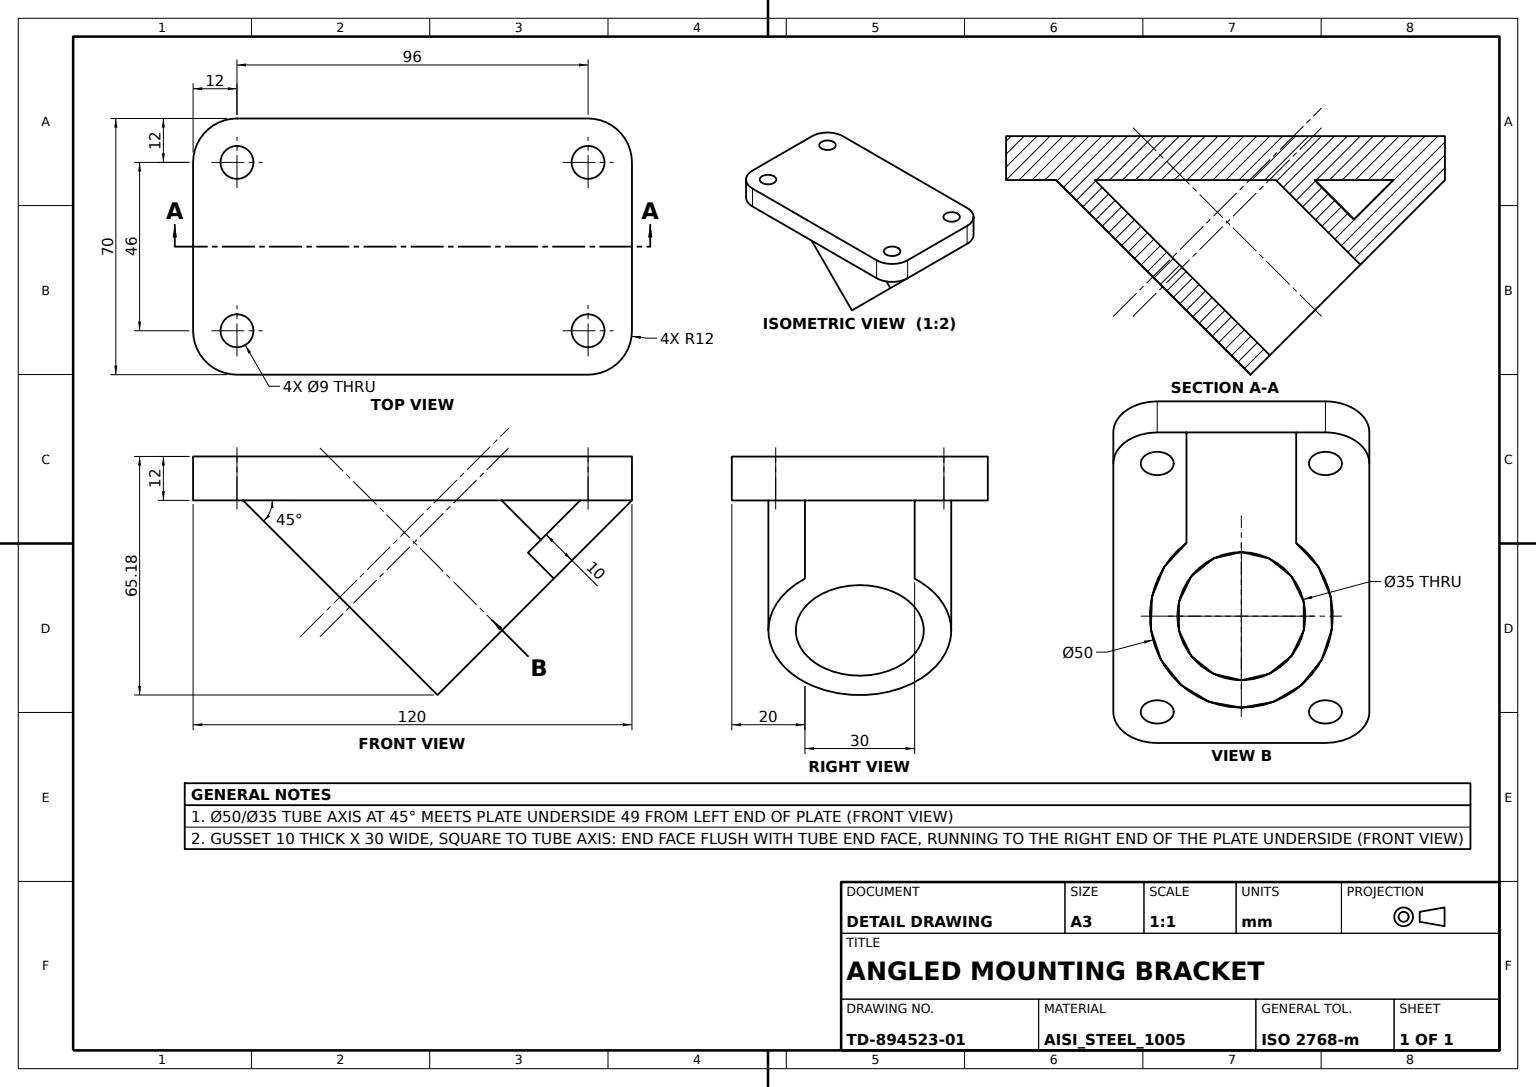
ISO-10303-21;
HEADER;
FILE_DESCRIPTION((''),'2;1');
FILE_NAME('','',(''),(''),'','','');
FILE_SCHEMA(('AUTOMOTIVE_DESIGN'));
ENDSEC;
DATA;
#1=APPLICATION_CONTEXT('');
#2=PRODUCT_CONTEXT('',#1,'mechanical');
#3=PRODUCT('','','',(#2));
#4=PRODUCT_DEFINITION_FORMATION('','',#3);
#5=PRODUCT_DEFINITION_CONTEXT('',#1,'design');
#6=PRODUCT_DEFINITION('','',#4,#5);
#7=PRODUCT_DEFINITION_SHAPE('','',#6);
#8=(LENGTH_UNIT()NAMED_UNIT(*)SI_UNIT(.MILLI.,.METRE.));
#9=(NAMED_UNIT(*)PLANE_ANGLE_UNIT()SI_UNIT($,.RADIAN.));
#10=(NAMED_UNIT(*)SI_UNIT($,.STERADIAN.)SOLID_ANGLE_UNIT());
#11=UNCERTAINTY_MEASURE_WITH_UNIT(LENGTH_MEASURE(0.005),#8,'distance_accuracy_value','');
#12=(GEOMETRIC_REPRESENTATION_CONTEXT(3)GLOBAL_UNCERTAINTY_ASSIGNED_CONTEXT((#11))GLOBAL_UNIT_ASSIGNED_CONTEXT((#8,#9,#10))REPRESENTATION_CONTEXT('',''));
#13=CARTESIAN_POINT('',(-50.,120.,0.));
#14=VERTEX_POINT('',#13);
#15=CARTESIAN_POINT('',(-50.,105.857864,0.));
#16=VERTEX_POINT('',#15);
#17=CARTESIAN_POINT('',(-50.,0.,0.));
#18=DIRECTION('',(0.,-1.,0.));
#19=VECTOR('',#18,1000.);
#20=LINE('',#17,#19);
#21=EDGE_CURVE('',#14,#16,#20,.T.);
#22=ORIENTED_EDGE('',*,*,#21,.F.);
#23=CARTESIAN_POINT('',(-50.,98.642136,-21.357864));
#24=VERTEX_POINT('',#23);
#25=DIRECTION('',(0.,-0.707106781,-0.707106781));
#26=VECTOR('',#25,1000.);
#27=LINE('',#13,#26);
#28=EDGE_CURVE('',#14,#24,#27,.T.);
#29=ORIENTED_EDGE('',*,*,#28,.T.);
#30=CARTESIAN_POINT('',(-50.,91.571068,-14.286797));
#31=VERTEX_POINT('',#30);
#32=CARTESIAN_POINT('',(-50.,26.042136,51.242136));
#33=DIRECTION('',(0.,0.707106781,-0.707106781));
#34=VECTOR('',#33,1000.);
#35=LINE('',#32,#34);
#36=EDGE_CURVE('',#31,#24,#35,.T.);
#37=ORIENTED_EDGE('',*,*,#36,.F.);
#38=CARTESIAN_POINT('',(-50.,112.928932,7.071068));
#39=LINE('',#38,#26);
#40=EDGE_CURVE('',#16,#31,#39,.T.);
#41=ORIENTED_EDGE('',*,*,#40,.F.);
#42=EDGE_LOOP('',(#22,#29,#37,#41));
#43=FACE_BOUND('',#42,.T.);
#44=DIRECTION('',(1.,0.,0.));
#45=DIRECTION('',(0.,0.,-1.));
#46=AXIS2_PLACEMENT_3D('',#38,#44,#45);
#47=PLANE('',#46);
#48=ADVANCED_FACE('',(#43),#47,.F.);
#49=CARTESIAN_POINT('',(-20.,120.,0.));
#50=VERTEX_POINT('',#49);
#51=DIRECTION('',(-1.,0.,0.));
#52=VECTOR('',#51,1000.);
#53=LINE('',#49,#52);
#54=EDGE_CURVE('',#50,#14,#53,.T.);
#55=ORIENTED_EDGE('',*,*,#54,.F.);
#56=CARTESIAN_POINT('',(-20.,98.642136,-21.357864));
#57=VERTEX_POINT('',#56);
#58=CARTESIAN_POINT('',(-20.,97.739823,-22.260177));
#59=DIRECTION('',(0.,0.707106781,0.707106781));
#60=VECTOR('',#59,1000.);
#61=LINE('',#58,#60);
#62=EDGE_CURVE('',#57,#50,#61,.T.);
#63=ORIENTED_EDGE('',*,*,#62,.F.);
#64=CARTESIAN_POINT('',(-35.,84.5,-35.5));
#65=AXIS2_PLACEMENT_3D('',#64,#33,#44);
#66=CIRCLE('',#65,25.);
#67=EDGE_CURVE('',#57,#24,#66,.T.);
#68=ORIENTED_EDGE('',*,*,#67,.T.);
#69=ORIENTED_EDGE('',*,*,#28,.F.);
#70=EDGE_LOOP('',(#55,#63,#68,#69));
#71=FACE_BOUND('',#70,.T.);
#72=CARTESIAN_POINT('',(-17.5,84.5,-35.5));
#73=VERTEX_POINT('',#72);
#74=CIRCLE('',#65,17.5);
#75=EDGE_CURVE('',#73,#73,#74,.T.);
#76=ORIENTED_EDGE('',*,*,#75,.F.);
#77=EDGE_LOOP('',(#76));
#78=FACE_BOUND('',#77,.T.);
#79=AXIS2_PLACEMENT_3D('',#64,#33,#59);
#80=PLANE('',#79);
#81=ADVANCED_FACE('',(#71,#78),#80,.T.);
#82=CARTESIAN_POINT('',(-20.,91.571068,-14.286797));
#83=VERTEX_POINT('',#82);
#84=CARTESIAN_POINT('',(-20.,105.857864,0.));
#85=VERTEX_POINT('',#84);
#86=CARTESIAN_POINT('',(-20.,90.668755,-15.18911));
#87=LINE('',#86,#60);
#88=EDGE_CURVE('',#83,#85,#87,.T.);
#89=ORIENTED_EDGE('',*,*,#88,.F.);
#90=CARTESIAN_POINT('',(-20.,26.042136,51.242136));
#91=LINE('',#90,#34);
#92=EDGE_CURVE('',#57,#83,#91,.F.);
#93=ORIENTED_EDGE('',*,*,#92,.F.);
#94=ORIENTED_EDGE('',*,*,#62,.T.);
#95=CARTESIAN_POINT('',(-20.,0.,0.));
#96=DIRECTION('',(0.,1.,0.));
#97=VECTOR('',#96,1000.);
#98=LINE('',#95,#97);
#99=EDGE_CURVE('',#85,#50,#98,.T.);
#100=ORIENTED_EDGE('',*,*,#99,.F.);
#101=EDGE_LOOP('',(#89,#93,#94,#100));
#102=FACE_BOUND('',#101,.T.);
#103=DIRECTION('',(0.,0.,1.));
#104=AXIS2_PLACEMENT_3D('',#86,#51,#103);
#105=PLANE('',#104);
#106=ADVANCED_FACE('',(#102),#105,.F.);
#107=CARTESIAN_POINT('',(-16.5,12.,12.));
#108=VERTEX_POINT('',#107);
#109=CARTESIAN_POINT('',(-12.,12.,12.));
#110=AXIS2_PLACEMENT_3D('',#109,#45,#51);
#111=CIRCLE('',#110,4.5);
#112=EDGE_CURVE('',#108,#108,#111,.T.);
#113=ORIENTED_EDGE('',*,*,#112,.T.);
#114=EDGE_LOOP('',(#113));
#115=FACE_BOUND('',#114,.T.);
#116=CARTESIAN_POINT('',(-16.5,108.,12.));
#117=VERTEX_POINT('',#116);
#118=CARTESIAN_POINT('',(-12.,108.,12.));
#119=AXIS2_PLACEMENT_3D('',#118,#45,#51);
#120=CIRCLE('',#119,4.5);
#121=EDGE_CURVE('',#117,#117,#120,.T.);
#122=ORIENTED_EDGE('',*,*,#121,.T.);
#123=EDGE_LOOP('',(#122));
#124=FACE_BOUND('',#123,.T.);
#125=CARTESIAN_POINT('',(-62.5,108.,12.));
#126=VERTEX_POINT('',#125);
#127=CARTESIAN_POINT('',(-58.,108.,12.));
#128=AXIS2_PLACEMENT_3D('',#127,#45,#51);
#129=CIRCLE('',#128,4.5);
#130=EDGE_CURVE('',#126,#126,#129,.T.);
#131=ORIENTED_EDGE('',*,*,#130,.T.);
#132=EDGE_LOOP('',(#131));
#133=FACE_BOUND('',#132,.T.);
#134=CARTESIAN_POINT('',(-62.5,12.,12.));
#135=VERTEX_POINT('',#134);
#136=CARTESIAN_POINT('',(-58.,12.,12.));
#137=AXIS2_PLACEMENT_3D('',#136,#45,#51);
#138=CIRCLE('',#137,4.5);
#139=EDGE_CURVE('',#135,#135,#138,.T.);
#140=ORIENTED_EDGE('',*,*,#139,.T.);
#141=EDGE_LOOP('',(#140));
#142=FACE_BOUND('',#141,.T.);
#143=CARTESIAN_POINT('',(-12.,0.,12.));
#144=VERTEX_POINT('',#143);
#145=CARTESIAN_POINT('',(0.,12.,12.));
#146=VERTEX_POINT('',#145);
#147=CIRCLE('',#110,12.);
#148=EDGE_CURVE('',#144,#146,#147,.F.);
#149=ORIENTED_EDGE('',*,*,#148,.T.);
#150=CARTESIAN_POINT('',(0.,108.,12.));
#151=VERTEX_POINT('',#150);
#152=CARTESIAN_POINT('',(0.,120.,12.));
#153=LINE('',#152,#19);
#154=EDGE_CURVE('',#151,#146,#153,.T.);
#155=ORIENTED_EDGE('',*,*,#154,.F.);
#156=CARTESIAN_POINT('',(-12.,120.,12.));
#157=VERTEX_POINT('',#156);
#158=CIRCLE('',#119,12.);
#159=EDGE_CURVE('',#151,#157,#158,.F.);
#160=ORIENTED_EDGE('',*,*,#159,.T.);
#161=CARTESIAN_POINT('',(-58.,120.,12.));
#162=VERTEX_POINT('',#161);
#163=CARTESIAN_POINT('',(-70.,120.,12.));
#164=VECTOR('',#44,1000.);
#165=LINE('',#163,#164);
#166=EDGE_CURVE('',#162,#157,#165,.T.);
#167=ORIENTED_EDGE('',*,*,#166,.F.);
#168=CARTESIAN_POINT('',(-70.,108.,12.));
#169=VERTEX_POINT('',#168);
#170=CIRCLE('',#128,12.);
#171=EDGE_CURVE('',#162,#169,#170,.F.);
#172=ORIENTED_EDGE('',*,*,#171,.T.);
#173=CARTESIAN_POINT('',(-70.,12.,12.));
#174=VERTEX_POINT('',#173);
#175=CARTESIAN_POINT('',(-70.,0.,12.));
#176=LINE('',#175,#97);
#177=EDGE_CURVE('',#174,#169,#176,.T.);
#178=ORIENTED_EDGE('',*,*,#177,.F.);
#179=CARTESIAN_POINT('',(-58.,0.,12.));
#180=VERTEX_POINT('',#179);
#181=CIRCLE('',#137,12.);
#182=EDGE_CURVE('',#174,#180,#181,.F.);
#183=ORIENTED_EDGE('',*,*,#182,.T.);
#184=CARTESIAN_POINT('',(0.,0.,12.));
#185=LINE('',#184,#52);
#186=EDGE_CURVE('',#144,#180,#185,.T.);
#187=ORIENTED_EDGE('',*,*,#186,.F.);
#188=EDGE_LOOP('',(#149,#155,#160,#167,#172,#178,#183,#187));
#189=FACE_BOUND('',#188,.T.);
#190=AXIS2_PLACEMENT_3D('',#184,#45,#51);
#191=PLANE('',#190);
#192=ADVANCED_FACE('',(#115,#124,#133,#142,#189),#191,.F.);
#193=CARTESIAN_POINT('',(-62.5,12.,0.));
#194=VERTEX_POINT('',#193);
#195=CARTESIAN_POINT('',(-58.,12.,0.));
#196=AXIS2_PLACEMENT_3D('',#195,#45,#51);
#197=CIRCLE('',#196,4.5);
#198=EDGE_CURVE('',#194,#194,#197,.T.);
#199=ORIENTED_EDGE('',*,*,#198,.T.);
#200=EDGE_LOOP('',(#199));
#201=FACE_BOUND('',#200,.T.);
#202=ORIENTED_EDGE('',*,*,#139,.F.);
#203=EDGE_LOOP('',(#202));
#204=FACE_BOUND('',#203,.T.);
#205=CYLINDRICAL_SURFACE('',#137,4.5);
#206=ADVANCED_FACE('',(#201,#204),#205,.F.);
#207=CARTESIAN_POINT('',(-70.,108.,0.));
#208=VERTEX_POINT('',#207);
#209=VECTOR('',#45,1000.);
#210=LINE('',#168,#209);
#211=EDGE_CURVE('',#169,#208,#210,.T.);
#212=ORIENTED_EDGE('',*,*,#211,.F.);
#213=ORIENTED_EDGE('',*,*,#171,.F.);
#214=CARTESIAN_POINT('',(-58.,120.,0.));
#215=VERTEX_POINT('',#214);
#216=LINE('',#161,#209);
#217=EDGE_CURVE('',#215,#162,#216,.F.);
#218=ORIENTED_EDGE('',*,*,#217,.F.);
#219=CARTESIAN_POINT('',(-58.,108.,0.));
#220=AXIS2_PLACEMENT_3D('',#219,#45,#51);
#221=CIRCLE('',#220,12.);
#222=EDGE_CURVE('',#208,#215,#221,.T.);
#223=ORIENTED_EDGE('',*,*,#222,.F.);
#224=EDGE_LOOP('',(#212,#213,#218,#223));
#225=FACE_BOUND('',#224,.T.);
#226=CYLINDRICAL_SURFACE('',#128,12.);
#227=ADVANCED_FACE('',(#225),#226,.T.);
#228=ORIENTED_EDGE('',*,*,#121,.F.);
#229=EDGE_LOOP('',(#228));
#230=FACE_BOUND('',#229,.T.);
#231=CARTESIAN_POINT('',(-16.5,108.,0.));
#232=VERTEX_POINT('',#231);
#233=CARTESIAN_POINT('',(-12.,108.,0.));
#234=AXIS2_PLACEMENT_3D('',#233,#45,#51);
#235=CIRCLE('',#234,4.5);
#236=EDGE_CURVE('',#232,#232,#235,.T.);
#237=ORIENTED_EDGE('',*,*,#236,.T.);
#238=EDGE_LOOP('',(#237));
#239=FACE_BOUND('',#238,.T.);
#240=CYLINDRICAL_SURFACE('',#119,4.5);
#241=ADVANCED_FACE('',(#230,#239),#240,.F.);
#242=CARTESIAN_POINT('',(-70.,12.,0.));
#243=VERTEX_POINT('',#242);
#244=LINE('',#173,#209);
#245=EDGE_CURVE('',#243,#174,#244,.F.);
#246=ORIENTED_EDGE('',*,*,#245,.T.);
#247=ORIENTED_EDGE('',*,*,#177,.T.);
#248=ORIENTED_EDGE('',*,*,#211,.T.);
#249=CARTESIAN_POINT('',(-70.,0.,0.));
#250=LINE('',#249,#97);
#251=EDGE_CURVE('',#243,#208,#250,.T.);
#252=ORIENTED_EDGE('',*,*,#251,.F.);
#253=EDGE_LOOP('',(#246,#247,#248,#252));
#254=FACE_BOUND('',#253,.T.);
#255=AXIS2_PLACEMENT_3D('',#175,#51,#103);
#256=PLANE('',#255);
#257=ADVANCED_FACE('',(#254),#256,.T.);
#258=CARTESIAN_POINT('',(-12.,0.,0.));
#259=VERTEX_POINT('',#258);
#260=CARTESIAN_POINT('',(-58.,0.,0.));
#261=VERTEX_POINT('',#260);
#262=CARTESIAN_POINT('',(0.,0.,0.));
#263=LINE('',#262,#52);
#264=EDGE_CURVE('',#259,#261,#263,.T.);
#265=ORIENTED_EDGE('',*,*,#264,.F.);
#266=LINE('',#143,#209);
#267=EDGE_CURVE('',#259,#144,#266,.F.);
#268=ORIENTED_EDGE('',*,*,#267,.T.);
#269=ORIENTED_EDGE('',*,*,#186,.T.);
#270=LINE('',#179,#209);
#271=EDGE_CURVE('',#180,#261,#270,.T.);
#272=ORIENTED_EDGE('',*,*,#271,.T.);
#273=EDGE_LOOP('',(#265,#268,#269,#272));
#274=FACE_BOUND('',#273,.T.);
#275=AXIS2_PLACEMENT_3D('',#184,#18,#44);
#276=PLANE('',#275);
#277=ADVANCED_FACE('',(#274),#276,.T.);
#278=ORIENTED_EDGE('',*,*,#75,.T.);
#279=EDGE_LOOP('',(#278));
#280=FACE_BOUND('',#279,.T.);
#281=CARTESIAN_POINT('',(-35.,73.748737,0.));
#282=VERTEX_POINT('',#281);
#283=CARTESIAN_POINT('',(-35.,49.,0.));
#284=AXIS2_PLACEMENT_3D('',#283,#45,#96);
#285=ELLIPSE('',#284,24.748737,17.5);
#286=EDGE_CURVE('',#282,#282,#285,.F.);
#287=ORIENTED_EDGE('',*,*,#286,.T.);
#288=EDGE_LOOP('',(#287));
#289=FACE_BOUND('',#288,.T.);
#290=CARTESIAN_POINT('',(-35.,11.9,37.1));
#291=AXIS2_PLACEMENT_3D('',#290,#33,#59);
#292=CYLINDRICAL_SURFACE('',#291,17.5);
#293=ADVANCED_FACE('',(#280,#289),#292,.F.);
#294=ORIENTED_EDGE('',*,*,#236,.F.);
#295=EDGE_LOOP('',(#294));
#296=FACE_BOUND('',#295,.T.);
#297=CARTESIAN_POINT('',(-62.5,108.,0.));
#298=VERTEX_POINT('',#297);
#299=CIRCLE('',#220,4.5);
#300=EDGE_CURVE('',#298,#298,#299,.T.);
#301=ORIENTED_EDGE('',*,*,#300,.F.);
#302=EDGE_LOOP('',(#301));
#303=FACE_BOUND('',#302,.T.);
#304=ORIENTED_EDGE('',*,*,#198,.F.);
#305=EDGE_LOOP('',(#304));
#306=FACE_BOUND('',#305,.T.);
#307=CARTESIAN_POINT('',(-35.,84.355339,0.));
#308=VERTEX_POINT('',#307);
#309=ELLIPSE('',#284,35.355339,25.);
#310=EDGE_CURVE('',#308,#308,#309,.F.);
#311=ORIENTED_EDGE('',*,*,#310,.T.);
#312=EDGE_LOOP('',(#311));
#313=FACE_BOUND('',#312,.T.);
#314=CARTESIAN_POINT('',(-12.,120.,0.));
#315=VERTEX_POINT('',#314);
#316=CARTESIAN_POINT('',(0.,108.,0.));
#317=VERTEX_POINT('',#316);
#318=CIRCLE('',#234,12.);
#319=EDGE_CURVE('',#315,#317,#318,.T.);
#320=ORIENTED_EDGE('',*,*,#319,.T.);
#321=CARTESIAN_POINT('',(0.,12.,0.));
#322=VERTEX_POINT('',#321);
#323=CARTESIAN_POINT('',(0.,120.,0.));
#324=LINE('',#323,#19);
#325=EDGE_CURVE('',#317,#322,#324,.T.);
#326=ORIENTED_EDGE('',*,*,#325,.T.);
#327=CARTESIAN_POINT('',(-12.,12.,0.));
#328=AXIS2_PLACEMENT_3D('',#327,#45,#51);
#329=CIRCLE('',#328,12.);
#330=EDGE_CURVE('',#322,#259,#329,.T.);
#331=ORIENTED_EDGE('',*,*,#330,.T.);
#332=ORIENTED_EDGE('',*,*,#264,.T.);
#333=CIRCLE('',#196,12.);
#334=EDGE_CURVE('',#261,#243,#333,.T.);
#335=ORIENTED_EDGE('',*,*,#334,.T.);
#336=ORIENTED_EDGE('',*,*,#251,.T.);
#337=ORIENTED_EDGE('',*,*,#222,.T.);
#338=CARTESIAN_POINT('',(-70.,120.,0.));
#339=LINE('',#338,#164);
#340=EDGE_CURVE('',#215,#14,#339,.T.);
#341=ORIENTED_EDGE('',*,*,#340,.T.);
#342=ORIENTED_EDGE('',*,*,#21,.T.);
#343=CARTESIAN_POINT('',(0.,105.857864,0.));
#344=LINE('',#343,#52);
#345=EDGE_CURVE('',#85,#16,#344,.T.);
#346=ORIENTED_EDGE('',*,*,#345,.F.);
#347=ORIENTED_EDGE('',*,*,#99,.T.);
#348=EDGE_CURVE('',#50,#315,#339,.T.);
#349=ORIENTED_EDGE('',*,*,#348,.T.);
#350=EDGE_LOOP('',(#320,#326,#331,#332,#335,#336,#337,#341,#342,#346,#347,#349));
#351=FACE_BOUND('',#350,.T.);
#352=CARTESIAN_POINT('',(-16.5,12.,0.));
#353=VERTEX_POINT('',#352);
#354=CIRCLE('',#328,4.5);
#355=EDGE_CURVE('',#353,#353,#354,.T.);
#356=ORIENTED_EDGE('',*,*,#355,.F.);
#357=EDGE_LOOP('',(#356));
#358=FACE_BOUND('',#357,.T.);
#359=AXIS2_PLACEMENT_3D('',#262,#45,#51);
#360=PLANE('',#359);
#361=ADVANCED_FACE('',(#296,#303,#306,#313,#351,#358),#360,.T.);
#362=LINE('',#156,#209);
#363=EDGE_CURVE('',#157,#315,#362,.T.);
#364=ORIENTED_EDGE('',*,*,#363,.F.);
#365=ORIENTED_EDGE('',*,*,#159,.F.);
#366=LINE('',#150,#209);
#367=EDGE_CURVE('',#317,#151,#366,.F.);
#368=ORIENTED_EDGE('',*,*,#367,.F.);
#369=ORIENTED_EDGE('',*,*,#319,.F.);
#370=EDGE_LOOP('',(#364,#365,#368,#369));
#371=FACE_BOUND('',#370,.T.);
#372=CYLINDRICAL_SURFACE('',#119,12.);
#373=ADVANCED_FACE('',(#371),#372,.T.);
#374=ORIENTED_EDGE('',*,*,#300,.T.);
#375=EDGE_LOOP('',(#374));
#376=FACE_BOUND('',#375,.T.);
#377=ORIENTED_EDGE('',*,*,#130,.F.);
#378=EDGE_LOOP('',(#377));
#379=FACE_BOUND('',#378,.T.);
#380=CYLINDRICAL_SURFACE('',#128,4.5);
#381=ADVANCED_FACE('',(#376,#379),#380,.F.);
#382=ORIENTED_EDGE('',*,*,#36,.T.);
#383=ORIENTED_EDGE('',*,*,#67,.F.);
#384=ORIENTED_EDGE('',*,*,#92,.T.);
#385=CARTESIAN_POINT('',(-35.,77.428932,-28.428932));
#386=DIRECTION('',(0.,-0.707106781,0.707106781));
#387=AXIS2_PLACEMENT_3D('',#385,#386,#25);
#388=CIRCLE('',#387,25.);
#389=EDGE_CURVE('',#31,#83,#388,.F.);
#390=ORIENTED_EDGE('',*,*,#389,.F.);
#391=EDGE_LOOP('',(#382,#383,#384,#390));
#392=FACE_BOUND('',#391,.T.);
#393=ORIENTED_EDGE('',*,*,#310,.F.);
#394=EDGE_LOOP('',(#393));
#395=FACE_BOUND('',#394,.T.);
#396=CYLINDRICAL_SURFACE('',#291,25.);
#397=ADVANCED_FACE('',(#392,#395),#396,.T.);
#398=ORIENTED_EDGE('',*,*,#267,.F.);
#399=ORIENTED_EDGE('',*,*,#330,.F.);
#400=LINE('',#145,#209);
#401=EDGE_CURVE('',#146,#322,#400,.T.);
#402=ORIENTED_EDGE('',*,*,#401,.F.);
#403=ORIENTED_EDGE('',*,*,#148,.F.);
#404=EDGE_LOOP('',(#398,#399,#402,#403));
#405=FACE_BOUND('',#404,.T.);
#406=CYLINDRICAL_SURFACE('',#110,12.);
#407=ADVANCED_FACE('',(#405),#406,.T.);
#408=ORIENTED_EDGE('',*,*,#182,.F.);
#409=ORIENTED_EDGE('',*,*,#245,.F.);
#410=ORIENTED_EDGE('',*,*,#334,.F.);
#411=ORIENTED_EDGE('',*,*,#271,.F.);
#412=EDGE_LOOP('',(#408,#409,#410,#411));
#413=FACE_BOUND('',#412,.T.);
#414=CYLINDRICAL_SURFACE('',#137,12.);
#415=ADVANCED_FACE('',(#413),#414,.T.);
#416=ORIENTED_EDGE('',*,*,#112,.F.);
#417=EDGE_LOOP('',(#416));
#418=FACE_BOUND('',#417,.T.);
#419=ORIENTED_EDGE('',*,*,#355,.T.);
#420=EDGE_LOOP('',(#419));
#421=FACE_BOUND('',#420,.T.);
#422=CYLINDRICAL_SURFACE('',#110,4.5);
#423=ADVANCED_FACE('',(#418,#421),#422,.F.);
#424=ORIENTED_EDGE('',*,*,#286,.F.);
#425=EDGE_LOOP('',(#424));
#426=FACE_BOUND('',#425,.T.);
#427=ADVANCED_FACE('',(#426),#360,.T.);
#428=ORIENTED_EDGE('',*,*,#40,.T.);
#429=ORIENTED_EDGE('',*,*,#389,.T.);
#430=ORIENTED_EDGE('',*,*,#88,.T.);
#431=ORIENTED_EDGE('',*,*,#345,.T.);
#432=EDGE_LOOP('',(#428,#429,#430,#431));
#433=FACE_BOUND('',#432,.T.);
#434=CARTESIAN_POINT('',(0.,52.928932,-52.928932));
#435=AXIS2_PLACEMENT_3D('',#434,#386,#25);
#436=PLANE('',#435);
#437=ADVANCED_FACE('',(#433),#436,.T.);
#438=ORIENTED_EDGE('',*,*,#363,.T.);
#439=ORIENTED_EDGE('',*,*,#348,.F.);
#440=ORIENTED_EDGE('',*,*,#54,.T.);
#441=ORIENTED_EDGE('',*,*,#340,.F.);
#442=ORIENTED_EDGE('',*,*,#217,.T.);
#443=ORIENTED_EDGE('',*,*,#166,.T.);
#444=EDGE_LOOP('',(#438,#439,#440,#441,#442,#443));
#445=FACE_BOUND('',#444,.T.);
#446=AXIS2_PLACEMENT_3D('',#163,#96,#51);
#447=PLANE('',#446);
#448=ADVANCED_FACE('',(#445),#447,.T.);
#449=ORIENTED_EDGE('',*,*,#367,.T.);
#450=ORIENTED_EDGE('',*,*,#154,.T.);
#451=ORIENTED_EDGE('',*,*,#401,.T.);
#452=ORIENTED_EDGE('',*,*,#325,.F.);
#453=EDGE_LOOP('',(#449,#450,#451,#452));
#454=FACE_BOUND('',#453,.T.);
#455=AXIS2_PLACEMENT_3D('',#152,#44,#45);
#456=PLANE('',#455);
#457=ADVANCED_FACE('',(#454),#456,.T.);
#458=CLOSED_SHELL('',(#48,#81,#106,#192,#206,#227,#241,#257,#277,#293,#361,#373,#381,#397,#407,#415,#423,#427,#437,#448,#457));
#459=MANIFOLD_SOLID_BREP('',#458);
#460=ADVANCED_BREP_SHAPE_REPRESENTATION('',(#459),#12);
#461=SHAPE_DEFINITION_REPRESENTATION(#7,#460);
ENDSEC;
END-ISO-10303-21;
